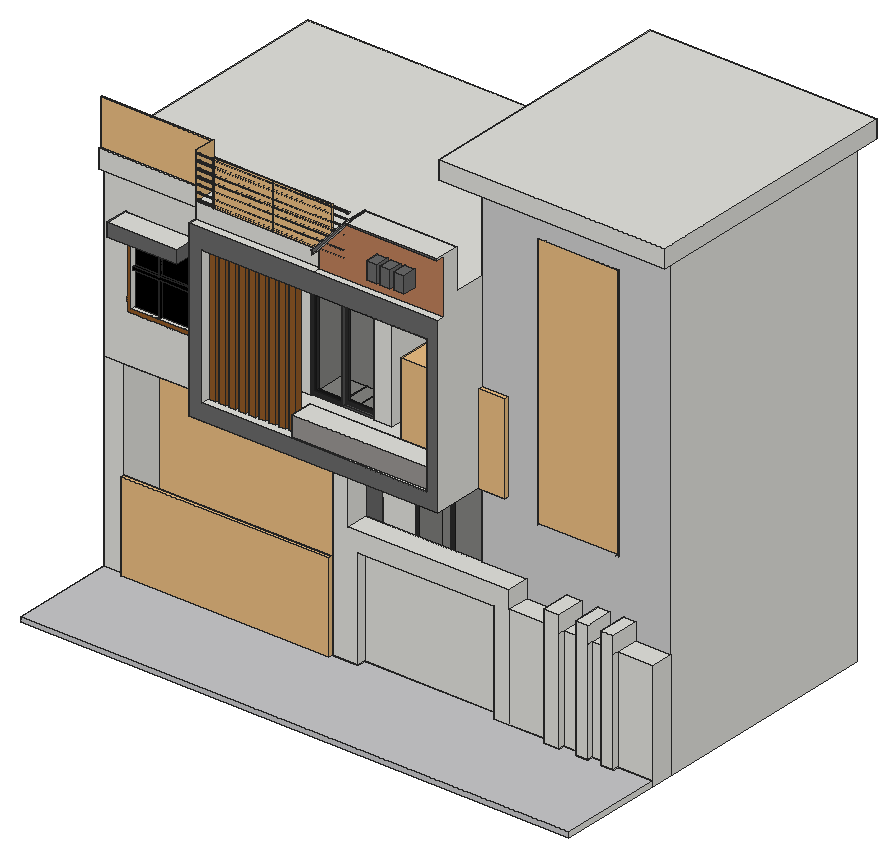
# SketchUp Ruby script. Lengths in inches.
U = 1.inch
M = Sketchup.active_model
def pt(a) = Geom::Point3d.new(a.map { |v| v * U })
def face(e, loops, mat)
  f = e.add_face(loops[0].map { |a| pt(a) })
  loops[1..].each { |l| e.add_face(l.map { |a| pt(a) }).erase! }
  f.material = f.back_material = mat if mat
  f
end
# faces: each face lists its corners as indices into pts; further lists are holes
def faces(e, pts, list, mat = nil) = list.each { |f| face(e, (f[0].is_a?(Array) ? f : [f]).map { |l| l.map { |i| pts[i] } }, mat) }
# xy, xz, yz: faces in a plane at the given z, y or x. An outline is a flat list of corners, or four numbers for a rectangle; further outlines are holes
def ring(l) = l.size == 4 ? [[l[0], l[1]], [l[2], l[1]], [l[2], l[3]], [l[0], l[3]]] : l.each_slice(2).to_a
def flat(e, list, mat, &to3) = list.each { |f| face(e, (f[0].is_a?(Array) ? f : [f]).map { |l| ring(l).map { |u, v| to3.(u, v) } }, mat) }
def xy(e, z, list, mat = nil) = flat(e, list, mat) { |x, y| [x, y, z] }
def xz(e, y, list, mat = nil) = flat(e, list, mat) { |x, z| [x, y, z] }
def yz(e, x, list, mat = nil) = flat(e, list, mat) { |y, z| [x, y, z] }
def lines(e, pts, list) = list.each { |a, b| e.add_line(pt(pts[a]), pt(pts[b])) }
# prism: a flat outline (further loops are holes) pulled along v
def prism(e, loops, v, mat = nil)
  f = face(e, loops, mat); d = Geom::Vector3d.new(v.map { |x| x * U })
  f.pushpull(f.normal.samedirection?(d) ? d.length : -d.length)
end
def box(e, o, s, mat = nil) = prism(e, [[o, [o[0] + s[0], o[1], o[2]], [o[0] + s[0], o[1] + s[1], o[2]], [o[0], o[1] + s[1], o[2]]]], [0, 0, s[2]], mat)
def at(x, y, z, deg = 0) = Geom::Transformation.translation(pt([x, y, z])) * Geom::Transformation.rotation(ORIGIN, Z_AXIS, deg.degrees)
def axes(o, x, y, z) = Geom::Transformation.new([*x, 0, *y, 0, *z, 0, *pt(o).to_a, 1])
def part(name) = M.definitions.add(name)
# library, detail: a bought-in or finely detailed component or shape, given as its bounding box
def library(name, o, s) = part(name).tap { |d| box(d.entities, o, s) }
def detail(e, o, s) = box(e.add_group.entities, o, s)
def put(e, d, t, mat = nil) = e.add_instance(d, t).tap { |i| i.material = mat if mat }
def group(e, t, mat = nil) = e.add_group.tap { |g| g.transformation = t; g.material = mat if mat }.entities
root = M.entities
M.materials.add("Glass_Tinted_Gray").color = [0, 0, 0]
M.materials["Glass_Tinted_Gray"].alpha = 0.125
M.materials.add("[0134_DimGray]").color = [105, 105, 105]
M.materials.add("[0135_DarkGray]").color = [81, 81, 81]
M.materials.add("[0137_Black]").color = [0, 0, 0]
M.materials.add("[Cladding Siding White]").color = [207, 207, 207]
M.materials.add("[Color A04]").color = [56, 56, 56]
M.materials.add("[Color_007]").color = [56, 56, 56]
M.materials.add("[Concrete Aggregate Smoke]").color = [154, 150, 148]
M.materials.add("[Mirror 02]").color = [229, 229, 229]
M.materials.add("[Polished Concrete New]").color = [200, 200, 203]
M.materials.add("[Terrazzo Light Blue]").color = [196, 214, 227]
M.materials.add("[Translucent_Glass_Gray]").color = [119, 126, 126]
M.materials["[Translucent_Glass_Gray]"].alpha = 0.2
M.materials.add("[Wood Cherry Original]").color = [152, 86, 42]
M.materials.add("[Wood Floor Parquet]").color = [145, 89, 39]
M.materials.add("[Wood Veneer 02]").color = [190, 128, 91]
c1 = library("Component\#72",[0,0,0],[1.18,52.35,94.49])
c2 = part("PENTEK_RP Fineline 50S_Sliding_DoorCase_E1")
box(c2.entities,[0,0,0],[1.51,3.66,99.27],"[0135_DarkGray]")
c3 = part("PENTEK_RP Fineline 50S_SlidingDooe_Case_E2")
box(c3.entities,[0,0,0],[96.25,3.66,1.51],"[0135_DarkGray]")
c4 = part("pentek_RP Fineline 50S_SlidingDoor_Case")
put(c4.entities,c2,at(97.76,0,0))
put(c4.entities,c3,at(1.51,0,0))
put(c4.entities,c2,at(0,0,0))
put(c4.entities,c3,at(1.51,0,97.76))
c5 = part("PENTEK_RP Fineline 50S_SlidingDoor_GlazingBead_2")
box(c5.entities,[0,0,0],[0.56,0.59,94.39],"[0135_DarkGray]")
c6 = part("PENTEK_RP Fineline 50S_SlidingDoor_Glass")
box(c6.entities,[0,0,0],[46.58,0.16,94.39],"Glass_Tinted_Gray")
c7 = part("PENTEK_RP Fineline 50S_SlidingDoor_GlazingBead")
box(c7.entities,[0,0,0],[45.47,0.59,0.56],"[0135_DarkGray]")
c8 = part("PENTEK_RP Fineline 50S_SlidingDoor_Leaf_E1")
xy(c8.entities,0,[[0,0,0.93,1.97],[0.93,1.57,1.49,1.97]],"[0135_DarkGray]")
xy(c8.entities,96.25,[[0,0,0.93,0,0.93,1.57,1.49,1.57,1.49,1.97,0,1.97]],"[0135_DarkGray]")
xz(c8.entities,0,[[0,0,0.93,96.25]],"[0135_DarkGray]")
xz(c8.entities,1.57,[[0.93,0,1.49,95.32],[0.93,95.32,1.49,96.25]],"[0135_DarkGray]")
xz(c8.entities,1.97,[[0,0,1.49,96.25]],"[0135_DarkGray]")
yz(c8.entities,0,[[0,0,1.97,96.25]],"[0135_DarkGray]")
yz(c8.entities,0.93,[[0,0,1.57,0.93],[0,0.93,1.57,95.32],[0,95.32,1.57,96.25]],"[0135_DarkGray]")
yz(c8.entities,1.49,[[1.57,0,1.97,95.32],[1.57,95.32,1.97,96.25]],"[0135_DarkGray]")
c9 = part("PENTEK_RP Fineline 50S_SlidingDoor_Leaf_E2")
xy(c9.entities,0,[[0,0,0,1.57,0.56,1.57,0.56,1.97,46.02,1.97,46.02,1.57,46.58,1.57,46.58,0]],"[0135_DarkGray]")
xy(c9.entities,0.93,[[0,0,46.58,1.57]],"[0135_DarkGray]")
xy(c9.entities,1.49,[[0.56,1.57,46.02,1.97]],"[0135_DarkGray]")
xz(c9.entities,0,[[0,0,46.58,0.93]],"[0135_DarkGray]")
xz(c9.entities,1.57,[[0,0,0.56,0.93],[46.02,0,46.58,0.93],[0.56,0.93,46.02,1.49]],"[0135_DarkGray]")
xz(c9.entities,1.97,[[0.56,0,46.02,1.49]],"[0135_DarkGray]")
yz(c9.entities,0,[[0,0,1.57,0.93]],"[0135_DarkGray]")
yz(c9.entities,0.56,[[1.57,0,1.97,0.93],[1.57,0.93,1.97,1.49]],"[0135_DarkGray]")
yz(c9.entities,46.02,[[1.57,0,1.97,0.93],[1.57,0.93,1.97,1.49]],"[0135_DarkGray]")
yz(c9.entities,46.58,[[0,0,1.57,0.93]],"[0135_DarkGray]")
c10 = part("PENTEK_RP Fineline S_SlidingDoor_Leaf1")
put(c10.entities,c5,at(0.93,0,0.93))
put(c10.entities,c5,at(46.96,0,0.93))
put(c10.entities,c6,at(1.49,1.42,0.93))
put(c10.entities,c7,at(1.49,0,0.93))
put(c10.entities,c6,at(1.49,0.59,0.93),"[Terrazzo Light Blue]")
put(c10.entities,c8,at(0,0,0))
put(c10.entities,c8,axes([48.44,0,0],[-1,0,0],[0,1,0],[0,0,1]))
put(c10.entities,c9,axes([0.93,0,96.25],[1,0,0],[0,1,0],[0,0,-1]))
put(c10.entities,c9,at(0.93,0,0))
put(c10.entities,c7,at(1.49,0,94.77))
c11 = part("PENTEK_RP Fineline 50S_SlidingDoor_Leaf2")
put(c11.entities,c6,at(1.49,1.42,0.93))
put(c11.entities,c7,at(1.49,0,94.77))
put(c11.entities,c5,at(46.96,0,0.93))
put(c11.entities,c6,at(1.49,0.59,0.93),"[Mirror 02]")
put(c11.entities,c5,at(0.93,0,0.93))
put(c11.entities,c8,at(0,0,0))
put(c11.entities,c8,axes([48.44,0,0],[-1,0,0],[0,1,0],[0,0,1]))
put(c11.entities,c7,at(1.49,0,0.93))
put(c11.entities,c9,axes([0.93,0,96.25],[1,0,0],[0,1,0],[0,0,-1]))
put(c11.entities,c9,at(0.93,0,0))
c12 = part("PENTEK - Slimmest Steel Sliding Door / Window\#1")
put(c12.entities,c4,at(0,-1.88,-0.09))
put(c12.entities,c10,at(1.51,-2.27,1.42))
put(c12.entities,c11,at(49.32,-0.3,1.42))
c13 = library("grille P1",[0,0,0],[0.79,28.9,72.83])
c14 = part("P1")
prism(c14.entities,[[[0.29,0.77,0],[0.39,0.79,0],[0.5,0.77,0],[0.59,0.73,0],[0.67,0.67,0],[0.73,0.59,0],[0.77,0.5,0],[0.79,0.39,0],[0.77,0.29,0],[0.73,0.2,0],[0.67,0.12,0],[0.59,0.05,0],[0.5,0.01,0],[0.39,0,0],[0.29,0.01,0],[0.2,0.05,0],[0.12,0.12,0],[0.05,0.2,0],[0.01,0.29,0],[0,0.39,0],[0.01,0.5,0],[0.05,0.59,0],[0.12,0.67,0],[0.2,0.73,0]]],[0,0,72.83])
p = [[0.39,0.39,0],[0.39,0.79,0]]
lines(c14.entities,p,[[0,1]])
c15 = part("bareau P1\#1")
prism(c15.entities,[[[0,27.72,7.875],[0,28.5,7.875],[0.79,28.5,7.875],[0.79,0,7.875],[0,0,7.875]]],[0,0,0.39])
p = [[0,27.72,0],[0,27.72,7.875],[0.39,27.72,0]]
lines(c15.entities,p,[[0,1],[2,0]])
c16 = part("bareau P1")
p = [[0.39,27.72,0],[0,27.72,0],[0.39,27.32,7.61],[0,27.32,7.61],[0.39,27.61,7.61],[0,1.78,-20.01],
  [0.79,1.78,-20.01],[0.39,28.25,7.875],[0.39,27.32,7.875]]
lines(c16.entities,p,[[0,1],[2,3],[2,4],[5,6],[7,8]])
detail(c16.entities,[0,0,-20.28],[0.79,28.9,28.55])
c17 = library("Achterdeur",[0,-0.05,0],[169.29,10.06,84.65])
c18 = part("Framed glazed panel")
g1 = group(c18.entities,at(1.97,102.36,3.69),"[Translucent_Glass_Gray]")
box(g1,[0,-21.65,-1.72],[0.94,35.43,108.27])
g2 = group(c18.entities,at(-1.97,0,-1.72),"[Color_007]")
g3 = group(g2,at(5.12,0,0),"[Color_007]")
prism(g3,[[[-3.15,78.74,1.72],[-3.15,78.74,113.93],[-3.15,120.08,113.93],[-3.15,120.08,1.72]],[[-3.15,118.11,111.96],[-3.15,80.71,111.96],[-3.15,80.71,3.69],[-3.15,118.11,3.69]]],[7.875,0,0])
g4 = group(g2,at(1.97,80.71,3.44),"[Color_007]")
prism(g4,[[[0,0,108.51],[0,37.4,108.51],[0,37.4,0.25],[0,0,0.25]],[[0,35.43,106.55],[0,1.97,106.55],[0,1.97,2.21],[0,35.43,2.21]]],[3.15,0,0])
c19 = library("plant",[-35.72,-28.42,0],[66.31,67.39,84.38])
c20 = library("Group\#3",[0,0,0],[39.37,8.78,82.68])
c21 = library("Group\#122",[0,0,0.875],[0.25,3.25,2.5])
c22 = library("Group\#5",[0,0,0],[107.6,5.33,60.06])
c23 = library("Group11\#2",[0.35,-39.08,0.31],[80.46,34.29,30.24])
xy(root,0,[[285.62,63.06,295.4,63.06,295.4,66.75,305.79,66.75,305.79,63.06,313.51,63.06,313.51,66.75,322.11,66.75,322.11,63.06,330.08,63.06,330.08,66.75,352.3125,66.75,352.3125,230.5,0,230.5,0,67.02,12.875,67.02,12.875,147.93,136.28,147.93,136.28,167.81,181.53,167.81,181.53,147.93,188.75,147.93,188.75,170.62,223.19,170.62,223.19,147.93,231.43,147.93,231.43,81.14,146.85,81.14,146.85,66.75,163.125,66.75,163.125,72.25,250.5625,72.25,250.5625,66.75,285.62,66.75],[12.875,66.75,12.875,67.02,0,67.02],[12.875,66.75,146.85,81.14],[[12.875,81.14,231.43,81.14,231.43,147.93,223.19,147.93,223.19,170.62,188.75,170.62,188.75,147.93,181.53,147.93,181.53,167.81,136.28,167.81,136.28,147.93,12.875,147.93],[133.52,95.32,142.33,112.41]]])
xy(root,3.3125,[[0,0,352.3125,0,352.3125,66.75,330.08,66.75,330.08,63.06,322.11,63.06,322.11,66.75,313.51,66.75,313.51,63.06,305.79,63.06,305.79,66.75,295.4,66.75,295.4,63.06,285.62,63.06,285.62,66.75,250.5625,66.75,250.5625,72.25,163.125,72.25,163.125,66.75,12.875,66.75,0,67.02]],"[Polished Concrete New]")
xy(root,68,[[163.125,66.75,250.5625,72.25]])
xy(root,69.5625,[[260.21,66.75,285.62,81.14],[295.4,66.75,305.79,81.14],[313.51,66.75,322.11,81.14],[330.08,66.75,352.3125,81.14]])
xy(root,80.625,[[285.62,63.06,295.4,81.14],[305.79,63.06,313.51,81.14],[322.11,63.06,330.08,81.14],[156.98,66.75,260.21,81.14]])
xy(root,81.75,[[136.28,147.93,181.53,167.81]])
xy(root,82.3125,[[188.75,147.93,223.19,170.62]])
xy(root,88.4,[[21.25,147.93,57.96,156.31]])
xy(root,111.08,[[21.25,147.93,57.96,156.31]])
xy(root,114.93,[[266.97,81.14,318.72,113.33]])
xy(root,123.94,[[71.58,45.77,71.58,67.02,12.875,67.02,12.875,147.93,231.43,147.93,231.43,45.77]])
xy(root,128.625,[[146.85,66.75,156.98,81.14]])
xy(root,133.94,[[79.99,45.77,224.4,45.77,224.4,47.48,136.52,47.48,136.52,61.89,224.4,61.89,224.4,153.46,216.32,153.46,216.32,204.9,181.69,204.9,181.69,153.46,169.04,153.46,169.04,86.65,157.4375,86.65,157.4375,110.83,142.33,110.83,142.33,95.32,133.52,95.32,133.52,110.83,116.9375,110.83,116.9375,86.65,79.99,86.65],[133.52,95.32,142.33,110.83],[133.52,110.83,142.33,112.41]])
xy(root,146.63,[[136.52,47.48,224.4,61.89]])
xy(root,156.98,[[17.25,67.02,54.86,89.71]])
xy(root,195.69,[[181.69,153.46,216.32,204.9]])
xy(root,199.47,[[116.9375,86.65,157.4375,110.83]])
xy(root,200.67,[[17.25,67.02,54.86,89.71]])
xy(root,203.36,[[13.8,52.52,58.3,67.02]])
xy(root,211.8,[[13.8,52.52,58.3,67.02]])
xy(root,221.91,[[79.99,45.77,79.99,86.65,169.04,86.65,169.04,153.46,224.4,153.46,224.4,45.77]])
xy(root,232.91,[[0,63.33,71.58,67.02]])
xy(root,234.49,[[71.58,45.77,151.5,51.58],[151.5,45.77,231.43,50.5]])
xy(root,245.05,[[188.6,41.89,195.22,50.5],[197.16,41.89,203.79,50.5],[206.1,41.89,212.72,50.5],[71.58,51.58,151.5,67.02],[151.5,60.77,231.43,60.77,231.43,230.5,0,230.5,0,63.33,71.58,63.33,71.58,67.02,151.5,67.02]])
xy(root,255.77,[[188.6,41.89,195.22,50.5],[197.16,41.89,203.79,50.5],[206.1,41.89,212.72,50.5]],"[0134_DimGray]")
xy(root,269.73,[[172.96,44.71,231.43,50.5]])
xy(root,270.61,[[173.23,44.71,231.43,60.77]])
xy(root,279.24,[[266.97,81.14,318.72,113.33]])
xy(root,304.8,[[219.87,60.64,352.3125,81.14],[352.3125,60.64,365,230.5],[219.87,81.14,231.43,230.5]],"[Wood Cherry Original]")
xy(root,316.5625,[[219.87,60.64,365,230.5]])
xz(root,0,[[0,0,352.3125,3.3125]],"[Polished Concrete New]")
xz(root,41.89,[[188.6,245.05,195.22,255.77],[197.16,245.05,203.79,255.77],[206.1,245.05,212.72,255.77]],"[0134_DimGray]")
xz(root,44.71,[[151.5,245.05,172.96,269.73,173.73,270.61,173.23,270.61,172.66,271.12,171.27,269.53,171.28,269.52,171.85,269.03,171.83,269.01,171.28,269.52,151.73,248.24,150.95,247.39,151.5,246.88],[172.96,269.73,231.43,269.73,231.43,270.61,173.73,270.61]],"[0134_DimGray]")
xz(root,45.77,[[[71.58,123.94,231.43,234.49],[79.99,133.94,224.4,221.91]]],"[0134_DimGray]")
xz(root,47.48,[[136.52,133.94,224.4,146.63]],"[Concrete Aggregate Smoke]")
xz(root,50.5,[[[151.5,234.49,231.43,234.49,231.43,269.73,172.96,269.73,151.5,245.05],[188.6,245.05,195.22,255.77],[197.16,245.05,203.79,255.77],[206.1,245.05,212.72,255.77]]],"[Wood Veneer 02]")
xz(root,51.58,[[71.58,234.49,151.5,245.05]])
xz(root,52.52,[[13.8,203.36,58.3,211.8]],"[0134_DimGray]")
xz(root,60.64,[[219.87,304.8,365,316.5625]])
xz(root,60.77,[[151.5,245.05,151.5,246.88,150.95,247.39,151.73,248.24,171.28,269.52,171.83,269.01,171.85,269.03,171.28,269.52,171.27,269.53,172.66,271.12,173.23,270.61,231.43,270.61,231.43,245.05]])
xz(root,61.89,[[136.52,133.94,224.4,146.63]])
xz(root,63.06,[[285.62,0,295.4,3.3125],[305.79,0,313.51,3.3125],[322.11,0,330.08,3.3125],[285.62,3.3125,295.4,80.625],[305.79,3.3125,313.51,80.625],
  [322.11,3.3125,330.08,80.625]])
xz(root,63.33,[[0,232.91,71.58,245.05]])
xz(root,66.75,[[12.875,0,146.85,3.3125],[146.85,0,163.125,3.3125],[250.5625,0,260.21,3.3125],[260.21,0,285.62,3.3125],[295.4,0,305.79,3.3125],
  [313.51,0,322.11,3.3125],[330.08,0,352.3125,3.3125],[146.85,3.3125,163.125,3.3125,163.125,68,250.5625,68,250.5625,3.3125,260.21,3.3125,260.21,80.625,156.98,80.625,156.98,128.625,146.85,128.625],[260.21,3.3125,285.62,69.5625],[295.4,3.3125,305.79,69.5625],
  [313.51,3.3125,322.11,69.5625],[330.08,3.3125,352.3125,69.5625]])
xz(root,67.02,[[0,0,12.875,123.94],[[0,123.94,71.58,232.91],[14.55,154.29,14.55,203.36,13.8,203.36,13.8,211.8,58.3,211.8,58.3,203.36,57.55,203.36,57.55,154.29]],[13.8,203.36,58.3,211.8]])
xz(root,67.02,[[[14.55,154.29,57.55,203.36],[17.25,156.98,54.86,200.67]]],"[Wood Floor Parquet]")
xz(root,72.25,[[163.125,0,250.5625,3.3125],[163.125,3.3125,250.5625,68]])
xz(root,81.14,[[146.85,0,146.85,128.625,156.98,128.625,156.98,80.625,231.43,80.625,231.43,0]])
xz(root,81.14,[[[260.21,69.5625,285.62,69.5625,285.62,80.625,295.4,80.625,295.4,69.5625,305.79,69.5625,305.79,80.625,313.51,80.625,313.51,69.5625,322.11,69.5625,322.11,80.625,330.08,80.625,330.08,69.5625,352.3125,69.5625,352.3125,304.8,231.43,304.8,231.43,80.625,260.21,80.625],[266.97,114.93,318.72,279.24]]],"[Cladding Siding White]")
xz(root,86.65,[[79.99,133.94,116.9375,133.94,116.9375,199.47,157.4375,199.47,157.4375,133.94,169.04,133.94,169.04,221.91,79.99,221.91]])
xz(root,89.71,[[17.25,156.98,54.86,200.67]])
xz(root,95.32,[[133.52,0,142.33,133.94]],"[0134_DimGray]")
xz(root,110.83,[[116.9375,133.94,157.4375,199.47]])
xz(root,112.41,[[133.52,0,142.33,133.94]])
xz(root,113.33,[[266.97,114.93,318.72,279.24]])
xz(root,147.93,[[[12.875,0,136.28,0,136.28,81.75,181.53,81.75,181.53,0,188.75,0,188.75,82.3125,223.19,82.3125,223.19,0,231.43,0,231.43,123.94,12.875,123.94],[21.25,88.4,57.96,111.08]]])
xz(root,153.46,[[169.04,133.94,181.69,133.94,181.69,195.69,216.32,195.69,216.32,133.94,224.4,133.94,224.4,221.91,169.04,221.91]])
xz(root,156.31,[[21.25,88.4,57.96,111.08]])
xz(root,167.81,[[136.28,0,181.53,81.75]])
xz(root,170.62,[[188.75,0,223.19,82.3125]])
xz(root,204.9,[[181.69,133.94,216.32,195.69]])
xz(root,230.5,[[0,0,12.875,245.05],[12.875,0,231.43,245.05],[231.43,0,231.43,304.8,219.87,304.8,219.87,316.5625,365,316.5625,365,304.8,352.3125,304.8,352.3125,0]])
yz(root,0,[[0,0,67.02,3.3125],[67.02,0,67.02,232.91,63.33,232.91,63.33,245.05,230.5,245.05,230.5,0]])
yz(root,12.875,[[67.02,0,147.93,123.94]])
yz(root,13.8,[[52.52,203.36,67.02,211.8]],"[0134_DimGray]")
yz(root,17.25,[[67.02,156.98,89.71,200.67]])
yz(root,21.25,[[147.93,88.4,156.31,111.08]])
yz(root,54.86,[[67.02,156.98,89.71,200.67]])
yz(root,57.96,[[147.93,88.4,156.31,111.08]])
yz(root,58.3,[[52.52,203.36,67.02,211.8]],"[0134_DimGray]")
yz(root,71.58,[[51.58,234.49,63.33,245.05]])
yz(root,71.58,[[45.77,123.94,67.02,140.07],[45.77,140.07,45.77,234.49,63.33,234.49,63.33,232.91,67.02,232.91,67.02,140.07]],"[0134_DimGray]")
yz(root,79.99,[[45.77,133.94,86.65,221.91]])
yz(root,116.9375,[[86.65,133.94,110.83,199.47]])
yz(root,133.52,[[95.32,0,112.41,133.94]],"[0134_DimGray]")
yz(root,136.28,[[147.93,0,167.81,81.75]])
yz(root,136.52,[[47.48,133.94,61.89,146.63]])
yz(root,142.33,[[95.32,0,112.41,133.94]],"[0134_DimGray]")
yz(root,146.85,[[66.75,0,81.14,128.625]])
yz(root,151.5,[[44.71,245.05,60.77,246.88]])
yz(root,151.5,[[50.5,234.49,51.58,245.05]],"[Wood Veneer 02]")
yz(root,156.98,[[66.75,80.625,81.14,128.625]])
yz(root,157.4375,[[86.65,133.94,110.83,199.47]])
yz(root,163.125,[[66.75,0,72.25,3.3125],[66.75,3.3125,72.25,68]])
yz(root,169.04,[[86.65,133.94,153.46,221.91]])
yz(root,181.53,[[147.93,0,167.81,81.75]])
yz(root,181.69,[[153.46,133.94,204.9,195.69]])
yz(root,188.6,[[41.89,245.05,50.5,255.77]],"[0134_DimGray]")
yz(root,188.75,[[147.93,0,170.62,82.3125]])
yz(root,195.22,[[41.89,245.05,50.5,255.77]],"[0134_DimGray]")
yz(root,197.16,[[41.89,245.05,50.5,255.77]],"[0134_DimGray]")
yz(root,203.79,[[41.89,245.05,50.5,255.77]],"[0134_DimGray]")
yz(root,206.1,[[41.89,245.05,50.5,255.77]],"[0134_DimGray]")
yz(root,212.72,[[41.89,245.05,50.5,255.77]],"[0134_DimGray]")
yz(root,216.32,[[153.46,133.94,204.9,195.69]])
yz(root,219.87,[[60.64,304.8,230.5,316.5625]])
yz(root,223.19,[[147.93,0,170.62,82.3125]])
yz(root,224.4,[[45.77,133.94,45.77,221.91,153.46,221.91,153.46,133.94,61.89,133.94,61.89,146.63,47.48,146.63,47.48,133.94]])
yz(root,231.43,[[81.14,0,147.93,123.94],[45.77,123.94,81.14,123.94,81.14,245.05,60.77,245.05,60.77,270.61,44.71,270.61,44.71,269.73,50.5,269.73,50.5,234.49,45.77,234.49],[81.14,245.05,230.5,304.8]])
yz(root,250.5625,[[66.75,0,72.25,3.3125],[66.75,3.3125,72.25,68]])
yz(root,260.21,[[66.75,69.5625,81.14,80.625]])
yz(root,266.97,[[81.14,114.93,113.33,279.24]])
yz(root,285.62,[[63.06,0,66.75,3.3125],[63.06,3.3125,66.75,69.5625],[63.06,69.5625,81.14,80.625]])
yz(root,295.4,[[63.06,0,66.75,3.3125],[63.06,3.3125,66.75,69.5625],[63.06,69.5625,81.14,80.625]])
yz(root,305.79,[[63.06,0,66.75,3.3125],[63.06,3.3125,66.75,69.5625],[63.06,69.5625,81.14,80.625]])
yz(root,313.51,[[63.06,0,66.75,3.3125],[63.06,3.3125,66.75,69.5625],[63.06,69.5625,81.14,80.625]])
yz(root,318.72,[[81.14,114.93,113.33,279.24]])
yz(root,322.11,[[63.06,0,66.75,3.3125],[63.06,3.3125,66.75,69.5625],[63.06,69.5625,81.14,80.625]])
yz(root,330.08,[[63.06,0,66.75,3.3125],[63.06,3.3125,66.75,69.5625],[63.06,69.5625,81.14,80.625]])
yz(root,352.3125,[[0,0,66.75,3.3125],[66.75,0,81.14,69.5625],[81.14,0,230.5,304.8]])
yz(root,365,[[60.64,304.8,230.5,316.5625]])
p = [[12.875,66.75,0],[0,67.02,0],[0,67.02,3.3125],[12.875,66.75,3.3125],[151.5,44.71,245.05],[151.5,50.5,245.05],
  [172.96,50.5,269.73],[172.96,44.71,269.73],[151.5,60.77,246.88],[151.5,44.71,246.88],[150.95,44.71,247.39],[150.95,60.77,247.39],
  [151.73,44.71,248.24],[151.73,60.77,248.24],[171.28,60.77,269.52],[171.28,44.71,269.52],[171.83,44.71,269.01],[171.83,60.77,269.01],
  [171.85,44.71,269.03],[171.85,60.77,269.03],[171.27,60.77,269.53],[171.27,44.71,269.53],[172.66,44.71,271.12],[172.66,60.77,271.12],
  [173.23,44.71,270.61],[173.23,60.77,270.61],[89.99,67.02,123.94],[89.99,67.02,133.94],[71.58,67.02,123.94],[79.99,67.02,140.07],
  [71.58,67.02,140.07],[224.4,205.21,0],[224.4,205.21,221.91],[200.68,230.5,0],[72.14,51.93,245.33],[72.14,52.42,245.33],
  [151.58,51.35,244.79],[167.6,51.58,263.56],[103.53,-475.63,467.82],[103.53,-478.98,467.82],[102.34,-478.98,467.82],[102.34,-475.63,467.82]]
faces(root,p,[[0,1,2,3],[4,5,6,7],[8,9,10,11],[10,12,13,11],[14,13,12,15],[16,17,14,15],[18,15,14,19],[16,18,19,17],
  [20,14,15,21],[21,22,23,20],[24,25,23,22]])
lines(root,p,[[26,27],[26,28],[29,30],[31,32],[33,31],[34,35],[36,37],[38,39],[39,40],[38,41]])
put(root,c1,axes([319.38,81.14,114.24],[0,1,0],[-1,0,0],[0,0,1.74625]))
put(root,c12,axes([117.17,89.81,134],[0.4056,0,0],[0,1.39217,0],[0,0,0.6622]))
put(root,c12,axes([135.63,148.78,0.08],[0.46238,0,0],[0,0.37589,0],[0,0,0.82349]))
put(root,c13,axes([0,65.32,245.05],[0,-1.28012,0],[0,0,1],[0.9827,0,0]))
put(root,c14,axes([72.14,51.4375,244.94],[0,1.24,0],[0,0,1],[1.33542,0,0]))
put(root,c14,axes([72.14,51.4375,249.42],[0,1.24,0],[0,0,1],[1.33542,0,0]))
put(root,c14,axes([72.14,51.4375,253.91],[0,1.24,0],[0,0,1],[1.33542,0,0]))
put(root,c14,axes([72.14,51.4375,258.4],[0,1.24,0],[0,0,1],[1.33542,0,0]))
put(root,c14,axes([72.14,51.4375,267.375],[0,1.24,0],[0,0,1],[1.33542,0,0]))
put(root,c14,axes([72.14,51.4375,271.86],[0,1.24,0],[0,0,1],[1.33542,0,0]))
put(root,c15,axes([72.14,51.4375,244.54],[0,1.24,0],[0,0,1],[1.33542,0,0]))
put(root,c16,axes([147.85,51.4375,244.54],[0,1.24,0],[0,0,1],[1.33542,0,0]))
put(root,c16,axes([109.73,51.4375,244.54],[0,1.24,0],[0,0,1],[1.33542,0,0]))
put(root,c14,axes([72.14,51.4375,262.89],[0,1.24,0],[0,0,1],[1.33542,0,0]))
put(root,c13,axes([71.4,65.32,245.15],[0.44864,0,0],[0,0,1],[0,-0.18857,0]))
put(root,c17,axes([11.42,95.39,-0.44],[0.72124,0,0],[0,1.48867,0],[0,0,1.46947]))
put(root,c18,axes([127.88,147.93,88.4],[0,0.29,0],[-0.88801,0,0],[0,0,0.2022]))
put(root,c19,axes([217.61,106.57,124.11],[1,0,0],[0,1,0],[0,0,0.68]))
g5 = group(root,at(79.99,51.34,133.94))
box(g5,[0,0,0],[4.49,4.29,92.01],"[Wood Floor Parquet]")
box(g5,[44.78,0,0],[4.48,4.29,92.01],"[Wood Floor Parquet]")
box(g5,[31.98,0,0],[4.49,4.29,92.01],"[Wood Floor Parquet]")
box(g5,[19.19,0,0],[4.49,4.29,92.01],"[Wood Floor Parquet]")
box(g5,[6.4,0,0],[4.48,4.29,92.01],"[Wood Floor Parquet]")
box(g5,[51.17,0,0],[4.49,4.29,92.01],"[Wood Floor Parquet]")
box(g5,[25.59,0,0],[4.48,4.29,92.01],"[Wood Floor Parquet]")
box(g5,[12.79,0,0],[4.49,4.29,92.01],"[Wood Floor Parquet]")
box(g5,[38.38,0,0],[4.49,4.29,92.01],"[Wood Floor Parquet]")
g6 = group(root,at(14.55,68.02,154.29))
xy(g6,0,[[0,0,0.77,4.28],[0.77,0,1.54,4.28],[1.54,0,40.13,4.28]],"[0137_Black]")
xy(g6,2.25,[[0.91,0,1.54,2.14],[1.54,0,19.68,2.14],[20.45,0,39.22,2.14],[0.91,2.14,19.68,4.28],[20.45,2.14,39.22,4.28]],"[0137_Black]")
xy(g6,24.875,[[0.91,0,19.68,2.14],[20.45,0,39.22,2.14],[0.91,2.14,19.68,4.28],[20.45,2.14,39.22,4.28]],"[0137_Black]")
xy(g6,26.79,[[0.91,0,19.68,2.14],[20.45,0,39.22,2.14],[0.91,2.14,19.68,4.28],[20.45,2.14,39.22,4.28]],"[0137_Black]")
xy(g6,49.42,[[0.91,0,19.68,2.14],[20.45,0,39.22,2.14],[0.91,2.14,19.68,4.28],[20.45,2.14,39.22,4.28]],"[0137_Black]")
xy(g6,51.66,[[0,0,40.13,4.28]],"[0137_Black]")
xz(g6,0,[[[0,0,40.13,51.66],[0.91,26.79,19.68,49.42],[0.91,2.25,19.68,24.875],[20.45,26.79,39.22,49.42],[20.45,2.25,39.22,24.875]]],"[0137_Black]")
xz(g6,2.14,[[0.91,2.25,19.68,24.875],[20.45,2.25,39.22,24.875],[0.91,26.79,19.68,49.42],[20.45,26.79,39.22,49.42]],"[0137_Black]")
xz(g6,4.28,[[[0,0,40.13,51.66],[0.91,26.79,19.68,49.42],[0.91,2.25,19.68,24.875],[20.45,26.79,39.22,49.42],[20.45,2.25,39.22,24.875]]],"[0137_Black]")
yz(g6,0,[[0,0,4.28,51.66]],"[0137_Black]")
yz(g6,0.91,[[0,2.25,2.14,24.875],[2.14,2.25,4.28,24.875],[0,26.79,2.14,49.42],[2.14,26.79,4.28,49.42]],"[0137_Black]")
yz(g6,19.68,[[0,2.25,2.14,24.875],[2.14,2.25,4.28,24.875],[0,26.79,2.14,49.42],[2.14,26.79,4.28,49.42]],"[0137_Black]")
yz(g6,20.45,[[0,2.25,2.14,24.875],[2.14,2.25,4.28,24.875],[0,26.79,2.14,49.42],[2.14,26.79,4.28,49.42]],"[0137_Black]")
yz(g6,39.22,[[0,2.25,2.14,24.875],[2.14,2.25,4.28,24.875],[0,26.79,2.14,49.42],[2.14,26.79,4.28,49.42]],"[0137_Black]")
yz(g6,40.13,[[0,0,4.28,51.66]],"[0137_Black]")
p = [[0.91,2.14,2.25],[0.77,2.14,2.25]]
lines(g6,p,[[0,1]])
put(root,c20,axes([181.69,153.46,133.94],[0.89984,0,0],[0,0.02127,0],[0,0,0.74688]))
put(root,c20,axes([188.75,147.93,0],[0.89984,0,0],[0,0.01812,0],[0,0,0.99559]))
put(root,c21,axes([-24.28,68.76,-25.39],[0.69147,0,0],[0,1,0],[0,0,1]),"[Color A04]")
put(root,c21,axes([-24.75,68.76,-25.39],[0.69147,0,0],[0,1,0],[0,0,1]),"[Color A04]")
put(root,c22,axes([12.875,66.75,0],[1.24,0,0],[0,-0.42,0],[0,0,1]))
put(root,c23,at(33.46,152.72,16.22),"[Wood Veneer 02]")
